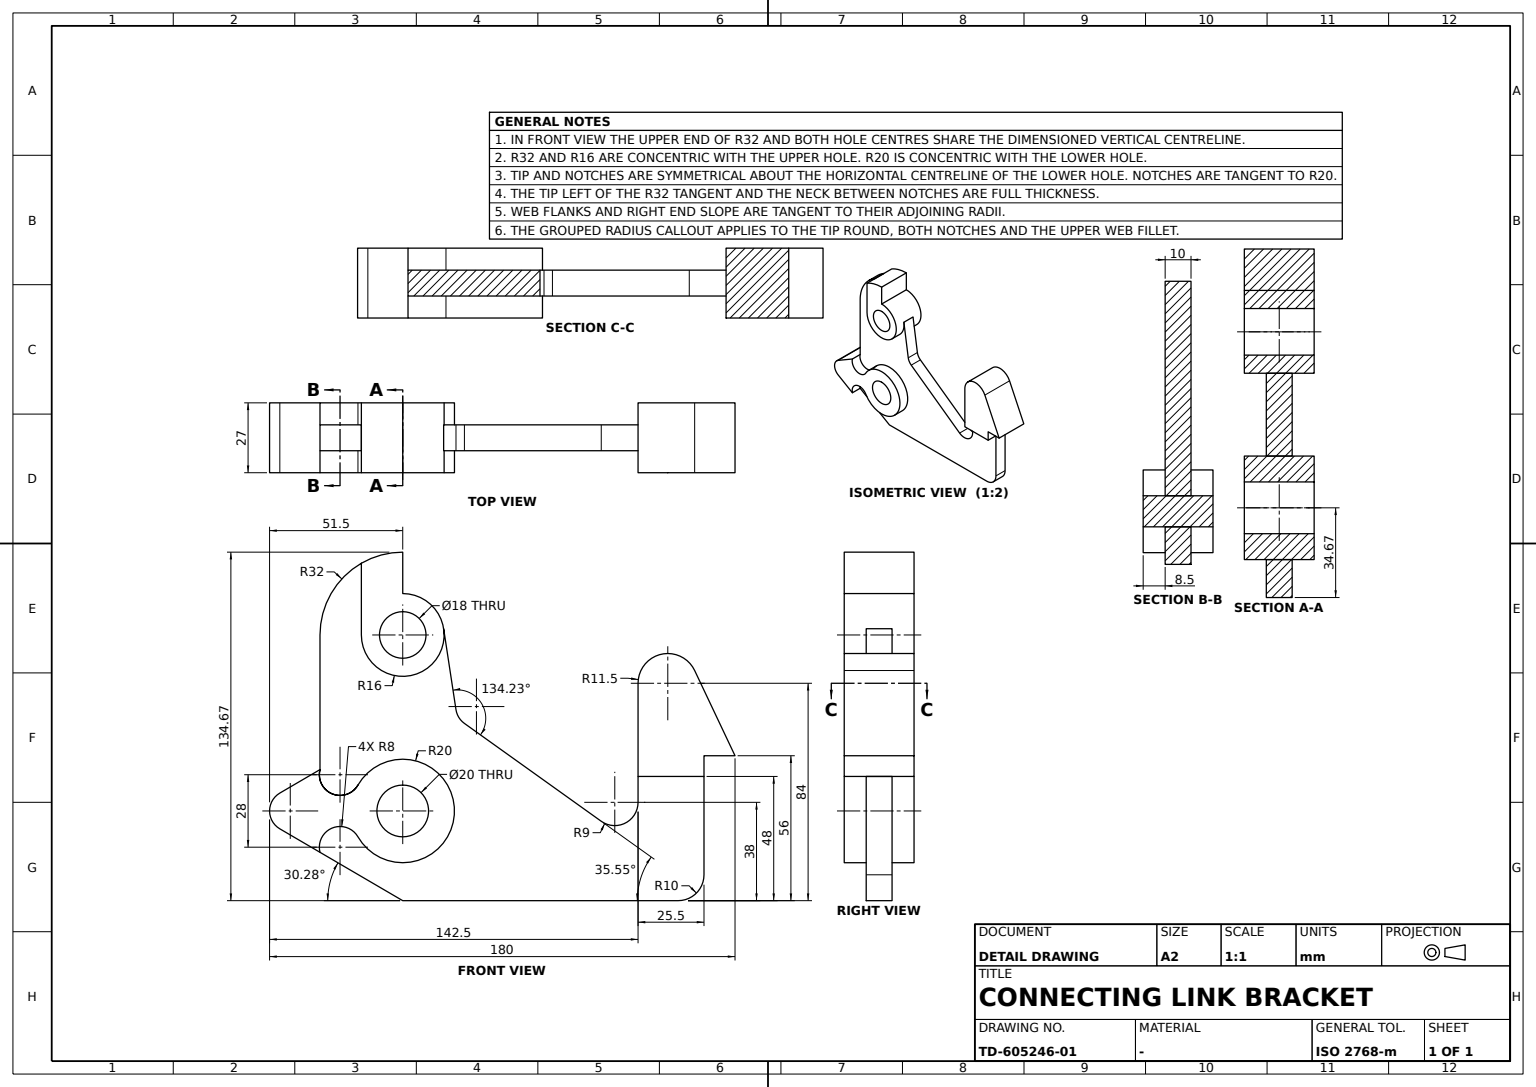
ISO-10303-21;
HEADER;
FILE_DESCRIPTION((''),'2;1');
FILE_NAME('','',(''),(''),'','','');
FILE_SCHEMA(('AUTOMOTIVE_DESIGN'));
ENDSEC;
DATA;
#1=APPLICATION_CONTEXT('');
#2=PRODUCT_CONTEXT('',#1,'mechanical');
#3=PRODUCT('','','',(#2));
#4=PRODUCT_DEFINITION_FORMATION('','',#3);
#5=PRODUCT_DEFINITION_CONTEXT('',#1,'design');
#6=PRODUCT_DEFINITION('','',#4,#5);
#7=PRODUCT_DEFINITION_SHAPE('','',#6);
#8=(LENGTH_UNIT()NAMED_UNIT(*)SI_UNIT(.MILLI.,.METRE.));
#9=(NAMED_UNIT(*)PLANE_ANGLE_UNIT()SI_UNIT($,.RADIAN.));
#10=(NAMED_UNIT(*)SI_UNIT($,.STERADIAN.)SOLID_ANGLE_UNIT());
#11=UNCERTAINTY_MEASURE_WITH_UNIT(LENGTH_MEASURE(0.005),#8,'distance_accuracy_value','');
#12=(GEOMETRIC_REPRESENTATION_CONTEXT(3)GLOBAL_UNCERTAINTY_ASSIGNED_CONTEXT((#11))GLOBAL_UNIT_ASSIGNED_CONTEXT((#8,#9,#10))REPRESENTATION_CONTEXT('',''));
#13=CARTESIAN_POINT('',(-32.,-5.,-15.979273));
#14=VERTEX_POINT('',#13);
#15=CARTESIAN_POINT('',(-32.,5.,-15.979273));
#16=VERTEX_POINT('',#15);
#17=DIRECTION('',(0.,1.,0.));
#18=VECTOR('',#17,1000.);
#19=LINE('',#13,#18);
#20=EDGE_CURVE('',#14,#16,#19,.T.);
#21=ORIENTED_EDGE('',*,*,#20,.T.);
#22=CARTESIAN_POINT('',(0.,5.,-34.665122));
#23=VERTEX_POINT('',#22);
#24=DIRECTION('',(0.863553516,0.,-0.504257201));
#25=VECTOR('',#24,1000.);
#26=LINE('',#15,#25);
#27=EDGE_CURVE('',#16,#23,#26,.T.);
#28=ORIENTED_EDGE('',*,*,#27,.T.);
#29=CARTESIAN_POINT('',(0.,-5.,-34.665122));
#30=VERTEX_POINT('',#29);
#31=LINE('',#29,#18);
#32=EDGE_CURVE('',#30,#23,#31,.T.);
#33=ORIENTED_EDGE('',*,*,#32,.F.);
#34=LINE('',#13,#25);
#35=EDGE_CURVE('',#14,#30,#34,.T.);
#36=ORIENTED_EDGE('',*,*,#35,.F.);
#37=EDGE_LOOP('',(#21,#28,#33,#36));
#38=FACE_BOUND('',#37,.T.);
#39=DIRECTION('',(0.504257201,0.,0.863553516));
#40=AXIS2_PLACEMENT_3D('',#13,#39,#24);
#41=PLANE('',#40);
#42=ADVANCED_FACE('',(#38),#41,.F.);
#43=CARTESIAN_POINT('',(20.591569,5.,39.127932));
#44=VERTEX_POINT('',#43);
#45=CARTESIAN_POINT('',(15.816862,5.,70.41389));
#46=VERTEX_POINT('',#45);
#47=DIRECTION('',(-0.150868155,0.,0.988553893));
#48=VECTOR('',#47,1000.);
#49=LINE('',#43,#48);
#50=EDGE_CURVE('',#44,#46,#49,.T.);
#51=ORIENTED_EDGE('',*,*,#50,.T.);
#52=CARTESIAN_POINT('',(15.816862,-5.,70.41389));
#53=VERTEX_POINT('',#52);
#54=LINE('',#52,#18);
#55=EDGE_CURVE('',#53,#46,#54,.T.);
#56=ORIENTED_EDGE('',*,*,#55,.F.);
#57=CARTESIAN_POINT('',(20.591569,-5.,39.127932));
#58=VERTEX_POINT('',#57);
#59=LINE('',#57,#48);
#60=EDGE_CURVE('',#58,#53,#59,.T.);
#61=ORIENTED_EDGE('',*,*,#60,.F.);
#62=LINE('',#57,#18);
#63=EDGE_CURVE('',#58,#44,#62,.T.);
#64=ORIENTED_EDGE('',*,*,#63,.T.);
#65=EDGE_LOOP('',(#51,#56,#61,#64));
#66=FACE_BOUND('',#65,.T.);
#67=DIRECTION('',(-0.988553893,0.,-0.150868155));
#68=AXIS2_PLACEMENT_3D('',#57,#67,#47);
#69=PLANE('',#68);
#70=ADVANCED_FACE('',(#66),#69,.F.);
#71=CARTESIAN_POINT('',(91.,-5.,3.334878));
#72=VERTEX_POINT('',#71);
#73=CARTESIAN_POINT('',(91.,5.,3.334878));
#74=VERTEX_POINT('',#73);
#75=LINE('',#71,#18);
#76=EDGE_CURVE('',#72,#74,#75,.T.);
#77=ORIENTED_EDGE('',*,*,#76,.F.);
#78=CARTESIAN_POINT('',(91.,-5.,13.334878));
#79=VERTEX_POINT('',#78);
#80=DIRECTION('',(0.,0.,-1.));
#81=VECTOR('',#80,1000.);
#82=LINE('',#78,#81);
#83=EDGE_CURVE('',#79,#72,#82,.T.);
#84=ORIENTED_EDGE('',*,*,#83,.F.);
#85=CARTESIAN_POINT('',(91.,5.,13.334878));
#86=VERTEX_POINT('',#85);
#87=LINE('',#78,#18);
#88=EDGE_CURVE('',#79,#86,#87,.T.);
#89=ORIENTED_EDGE('',*,*,#88,.T.);
#90=LINE('',#85,#81);
#91=EDGE_CURVE('',#86,#74,#90,.T.);
#92=ORIENTED_EDGE('',*,*,#91,.T.);
#93=EDGE_LOOP('',(#77,#84,#89,#92));
#94=FACE_BOUND('',#93,.T.);
#95=DIRECTION('',(1.,0.,0.));
#96=AXIS2_PLACEMENT_3D('',#78,#95,#80);
#97=PLANE('',#96);
#98=ADVANCED_FACE('',(#94),#97,.F.);
#99=CARTESIAN_POINT('',(0.,-5.,-20.));
#100=VERTEX_POINT('',#99);
#101=CARTESIAN_POINT('',(-17.320508,-5.,-10.));
#102=VERTEX_POINT('',#101);
#103=CARTESIAN_POINT('',(0.,-5.,0.));
#104=AXIS2_PLACEMENT_3D('',#103,#17,#95);
#105=CIRCLE('',#104,20.);
#106=EDGE_CURVE('',#100,#102,#105,.T.);
#107=ORIENTED_EDGE('',*,*,#106,.F.);
#108=CARTESIAN_POINT('',(0.,5.,-20.));
#109=VERTEX_POINT('',#108);
#110=LINE('',#99,#18);
#111=EDGE_CURVE('',#100,#109,#110,.T.);
#112=ORIENTED_EDGE('',*,*,#111,.T.);
#113=CARTESIAN_POINT('',(-17.320508,5.,-10.));
#114=VERTEX_POINT('',#113);
#115=CARTESIAN_POINT('',(0.,5.,0.));
#116=AXIS2_PLACEMENT_3D('',#115,#17,#95);
#117=CIRCLE('',#116,20.);
#118=EDGE_CURVE('',#109,#114,#117,.T.);
#119=ORIENTED_EDGE('',*,*,#118,.T.);
#120=LINE('',#101,#18);
#121=EDGE_CURVE('',#102,#114,#120,.T.);
#122=ORIENTED_EDGE('',*,*,#121,.F.);
#123=EDGE_LOOP('',(#107,#112,#119,#122));
#124=FACE_BOUND('',#123,.T.);
#125=DIRECTION('',(0.,0.,1.));
#126=AXIS2_PLACEMENT_3D('',#103,#17,#125);
#127=CYLINDRICAL_SURFACE('',#126,20.);
#128=ADVANCED_FACE('',(#124),#127,.F.);
#129=ORIENTED_EDGE('',*,*,#55,.T.);
#130=CARTESIAN_POINT('',(-16.,5.,68.));
#131=VERTEX_POINT('',#130);
#132=CARTESIAN_POINT('',(0.,5.,68.));
#133=AXIS2_PLACEMENT_3D('',#132,#17,#95);
#134=CIRCLE('',#133,16.);
#135=EDGE_CURVE('',#46,#131,#134,.T.);
#136=ORIENTED_EDGE('',*,*,#135,.T.);
#137=CARTESIAN_POINT('',(-16.,-5.,68.));
#138=VERTEX_POINT('',#137);
#139=LINE('',#137,#18);
#140=EDGE_CURVE('',#138,#131,#139,.T.);
#141=ORIENTED_EDGE('',*,*,#140,.F.);
#142=CARTESIAN_POINT('',(0.,-5.,68.));
#143=AXIS2_PLACEMENT_3D('',#142,#17,#95);
#144=CIRCLE('',#143,16.);
#145=EDGE_CURVE('',#53,#138,#144,.T.);
#146=ORIENTED_EDGE('',*,*,#145,.F.);
#147=EDGE_LOOP('',(#129,#136,#141,#146));
#148=FACE_BOUND('',#147,.T.);
#149=AXIS2_PLACEMENT_3D('',#142,#17,#125);
#150=CYLINDRICAL_SURFACE('',#149,16.);
#151=ADVANCED_FACE('',(#148),#150,.F.);
#152=CARTESIAN_POINT('',(23.848904,-5.,33.82586));
#153=VERTEX_POINT('',#152);
#154=CARTESIAN_POINT('',(23.848904,5.,33.82586));
#155=VERTEX_POINT('',#154);
#156=LINE('',#152,#18);
#157=EDGE_CURVE('',#153,#155,#156,.T.);
#158=ORIENTED_EDGE('',*,*,#157,.F.);
#159=CARTESIAN_POINT('',(76.767517,-5.,-3.987767));
#160=VERTEX_POINT('',#159);
#161=DIRECTION('',(-0.813627157,0.,0.581387005));
#162=VECTOR('',#161,1000.);
#163=LINE('',#159,#162);
#164=EDGE_CURVE('',#160,#153,#163,.T.);
#165=ORIENTED_EDGE('',*,*,#164,.F.);
#166=CARTESIAN_POINT('',(76.767517,5.,-3.987767));
#167=VERTEX_POINT('',#166);
#168=LINE('',#159,#18);
#169=EDGE_CURVE('',#160,#167,#168,.T.);
#170=ORIENTED_EDGE('',*,*,#169,.T.);
#171=LINE('',#166,#162);
#172=EDGE_CURVE('',#167,#155,#171,.T.);
#173=ORIENTED_EDGE('',*,*,#172,.T.);
#174=EDGE_LOOP('',(#158,#165,#170,#173));
#175=FACE_BOUND('',#174,.T.);
#176=DIRECTION('',(-0.581387005,0.,-0.813627157));
#177=AXIS2_PLACEMENT_3D('',#159,#176,#161);
#178=PLANE('',#177);
#179=ADVANCED_FACE('',(#175),#178,.F.);
#180=CARTESIAN_POINT('',(-16.,5.,95.712813));
#181=VERTEX_POINT('',#180);
#182=VECTOR('',#125,1000.);
#183=LINE('',#130,#182);
#184=EDGE_CURVE('',#131,#181,#183,.T.);
#185=ORIENTED_EDGE('',*,*,#184,.T.);
#186=CARTESIAN_POINT('',(-16.,-5.,95.712813));
#187=VERTEX_POINT('',#186);
#188=LINE('',#186,#18);
#189=EDGE_CURVE('',#187,#181,#188,.T.);
#190=ORIENTED_EDGE('',*,*,#189,.F.);
#191=LINE('',#137,#182);
#192=EDGE_CURVE('',#138,#187,#191,.T.);
#193=ORIENTED_EDGE('',*,*,#192,.F.);
#194=ORIENTED_EDGE('',*,*,#140,.T.);
#195=EDGE_LOOP('',(#185,#190,#193,#194));
#196=FACE_BOUND('',#195,.T.);
#197=DIRECTION('',(-1.,0.,0.));
#198=AXIS2_PLACEMENT_3D('',#137,#197,#125);
#199=PLANE('',#198);
#200=ADVANCED_FACE('',(#196),#199,.F.);
#201=CARTESIAN_POINT('',(-24.248711,-5.,-6.));
#202=VERTEX_POINT('',#201);
#203=CARTESIAN_POINT('',(-24.248711,5.,-6.));
#204=VERTEX_POINT('',#203);
#205=LINE('',#201,#18);
#206=EDGE_CURVE('',#202,#204,#205,.T.);
#207=ORIENTED_EDGE('',*,*,#206,.F.);
#208=CARTESIAN_POINT('',(-24.248711,-5.,-14.));
#209=DIRECTION('',(0.,-1.,0.));
#210=AXIS2_PLACEMENT_3D('',#208,#209,#95);
#211=CIRCLE('',#210,8.);
#212=EDGE_CURVE('',#102,#202,#211,.T.);
#213=ORIENTED_EDGE('',*,*,#212,.F.);
#214=ORIENTED_EDGE('',*,*,#121,.T.);
#215=CARTESIAN_POINT('',(-24.248711,5.,-14.));
#216=AXIS2_PLACEMENT_3D('',#215,#209,#95);
#217=CIRCLE('',#216,8.);
#218=EDGE_CURVE('',#114,#204,#217,.T.);
#219=ORIENTED_EDGE('',*,*,#218,.T.);
#220=EDGE_LOOP('',(#207,#213,#214,#219));
#221=FACE_BOUND('',#220,.T.);
#222=AXIS2_PLACEMENT_3D('',#208,#17,#125);
#223=CYLINDRICAL_SURFACE('',#222,8.);
#224=ADVANCED_FACE('',(#221),#223,.T.);
#225=CARTESIAN_POINT('',(-32.,-5.,15.979273));
#226=VERTEX_POINT('',#225);
#227=CARTESIAN_POINT('',(-32.,5.,15.979273));
#228=VERTEX_POINT('',#227);
#229=LINE('',#225,#18);
#230=EDGE_CURVE('',#226,#228,#229,.T.);
#231=ORIENTED_EDGE('',*,*,#230,.F.);
#232=CARTESIAN_POINT('',(-32.,-5.,68.));
#233=VERTEX_POINT('',#232);
#234=LINE('',#232,#81);
#235=EDGE_CURVE('',#233,#226,#234,.T.);
#236=ORIENTED_EDGE('',*,*,#235,.F.);
#237=CARTESIAN_POINT('',(-32.,5.,68.));
#238=VERTEX_POINT('',#237);
#239=LINE('',#232,#18);
#240=EDGE_CURVE('',#233,#238,#239,.T.);
#241=ORIENTED_EDGE('',*,*,#240,.T.);
#242=LINE('',#237,#81);
#243=EDGE_CURVE('',#238,#228,#242,.T.);
#244=ORIENTED_EDGE('',*,*,#243,.T.);
#245=EDGE_LOOP('',(#231,#236,#241,#244));
#246=FACE_BOUND('',#245,.T.);
#247=AXIS2_PLACEMENT_3D('',#232,#95,#80);
#248=PLANE('',#247);
#249=ADVANCED_FACE('',(#246),#248,.F.);
#250=CARTESIAN_POINT('',(-17.320508,-5.,10.));
#251=VERTEX_POINT('',#250);
#252=CARTESIAN_POINT('',(-24.248711,-5.,14.));
#253=AXIS2_PLACEMENT_3D('',#252,#209,#95);
#254=CIRCLE('',#253,8.);
#255=EDGE_CURVE('',#226,#251,#254,.T.);
#256=ORIENTED_EDGE('',*,*,#255,.F.);
#257=ORIENTED_EDGE('',*,*,#230,.T.);
#258=CARTESIAN_POINT('',(-17.320508,5.,10.));
#259=VERTEX_POINT('',#258);
#260=CARTESIAN_POINT('',(-24.248711,5.,14.));
#261=AXIS2_PLACEMENT_3D('',#260,#209,#95);
#262=CIRCLE('',#261,8.);
#263=EDGE_CURVE('',#228,#259,#262,.T.);
#264=ORIENTED_EDGE('',*,*,#263,.T.);
#265=LINE('',#250,#18);
#266=EDGE_CURVE('',#251,#259,#265,.T.);
#267=ORIENTED_EDGE('',*,*,#266,.F.);
#268=EDGE_LOOP('',(#256,#257,#264,#267));
#269=FACE_BOUND('',#268,.T.);
#270=AXIS2_PLACEMENT_3D('',#252,#17,#125);
#271=CYLINDRICAL_SURFACE('',#270,8.);
#272=ADVANCED_FACE('',(#269),#271,.T.);
#273=ORIENTED_EDGE('',*,*,#157,.T.);
#274=CARTESIAN_POINT('',(28.5,5.,40.334878));
#275=AXIS2_PLACEMENT_3D('',#274,#17,#95);
#276=CIRCLE('',#275,8.);
#277=EDGE_CURVE('',#155,#44,#276,.T.);
#278=ORIENTED_EDGE('',*,*,#277,.T.);
#279=ORIENTED_EDGE('',*,*,#63,.F.);
#280=CARTESIAN_POINT('',(28.5,-5.,40.334878));
#281=AXIS2_PLACEMENT_3D('',#280,#17,#95);
#282=CIRCLE('',#281,8.);
#283=EDGE_CURVE('',#153,#58,#282,.T.);
#284=ORIENTED_EDGE('',*,*,#283,.F.);
#285=EDGE_LOOP('',(#273,#278,#279,#284));
#286=FACE_BOUND('',#285,.T.);
#287=AXIS2_PLACEMENT_3D('',#280,#17,#125);
#288=CYLINDRICAL_SURFACE('',#287,8.);
#289=ADVANCED_FACE('',(#286),#288,.F.);
#290=ORIENTED_EDGE('',*,*,#240,.F.);
#291=AXIS2_PLACEMENT_3D('',#142,#209,#95);
#292=CIRCLE('',#291,32.);
#293=EDGE_CURVE('',#187,#233,#292,.T.);
#294=ORIENTED_EDGE('',*,*,#293,.F.);
#295=ORIENTED_EDGE('',*,*,#189,.T.);
#296=AXIS2_PLACEMENT_3D('',#132,#209,#95);
#297=CIRCLE('',#296,32.);
#298=EDGE_CURVE('',#181,#238,#297,.T.);
#299=ORIENTED_EDGE('',*,*,#298,.T.);
#300=EDGE_LOOP('',(#290,#294,#295,#299));
#301=FACE_BOUND('',#300,.T.);
#302=CYLINDRICAL_SURFACE('',#149,32.);
#303=ADVANCED_FACE('',(#301),#302,.T.);
#304=CARTESIAN_POINT('',(116.5,-5.,13.334878));
#305=VERTEX_POINT('',#304);
#306=CARTESIAN_POINT('',(116.5,5.,13.334878));
#307=VERTEX_POINT('',#306);
#308=LINE('',#304,#18);
#309=EDGE_CURVE('',#305,#307,#308,.T.);
#310=ORIENTED_EDGE('',*,*,#309,.F.);
#311=CARTESIAN_POINT('',(116.5,-5.,-24.665122));
#312=VERTEX_POINT('',#311);
#313=LINE('',#311,#182);
#314=EDGE_CURVE('',#312,#305,#313,.T.);
#315=ORIENTED_EDGE('',*,*,#314,.F.);
#316=CARTESIAN_POINT('',(116.5,5.,-24.665122));
#317=VERTEX_POINT('',#316);
#318=LINE('',#311,#18);
#319=EDGE_CURVE('',#312,#317,#318,.T.);
#320=ORIENTED_EDGE('',*,*,#319,.T.);
#321=LINE('',#316,#182);
#322=EDGE_CURVE('',#317,#307,#321,.T.);
#323=ORIENTED_EDGE('',*,*,#322,.T.);
#324=EDGE_LOOP('',(#310,#315,#320,#323));
#325=FACE_BOUND('',#324,.T.);
#326=AXIS2_PLACEMENT_3D('',#311,#197,#125);
#327=PLANE('',#326);
#328=ADVANCED_FACE('',(#325),#327,.F.);
#329=ORIENTED_EDGE('',*,*,#32,.T.);
#330=CARTESIAN_POINT('',(106.5,5.,-34.665122));
#331=VERTEX_POINT('',#330);
#332=VECTOR('',#95,1000.);
#333=LINE('',#22,#332);
#334=EDGE_CURVE('',#23,#331,#333,.T.);
#335=ORIENTED_EDGE('',*,*,#334,.T.);
#336=CARTESIAN_POINT('',(106.5,-5.,-34.665122));
#337=VERTEX_POINT('',#336);
#338=LINE('',#336,#18);
#339=EDGE_CURVE('',#337,#331,#338,.T.);
#340=ORIENTED_EDGE('',*,*,#339,.F.);
#341=LINE('',#29,#332);
#342=EDGE_CURVE('',#30,#337,#341,.T.);
#343=ORIENTED_EDGE('',*,*,#342,.F.);
#344=EDGE_LOOP('',(#329,#335,#340,#343));
#345=FACE_BOUND('',#344,.T.);
#346=AXIS2_PLACEMENT_3D('',#29,#125,#95);
#347=PLANE('',#346);
#348=ADVANCED_FACE('',(#345),#347,.F.);
#349=ORIENTED_EDGE('',*,*,#135,.F.);
#350=ORIENTED_EDGE('',*,*,#50,.F.);
#351=ORIENTED_EDGE('',*,*,#277,.F.);
#352=ORIENTED_EDGE('',*,*,#172,.F.);
#353=CARTESIAN_POINT('',(82.,5.,3.334878));
#354=AXIS2_PLACEMENT_3D('',#353,#17,#95);
#355=CIRCLE('',#354,9.);
#356=EDGE_CURVE('',#74,#167,#355,.T.);
#357=ORIENTED_EDGE('',*,*,#356,.F.);
#358=ORIENTED_EDGE('',*,*,#91,.F.);
#359=VECTOR('',#197,1000.);
#360=LINE('',#306,#359);
#361=EDGE_CURVE('',#307,#86,#360,.T.);
#362=ORIENTED_EDGE('',*,*,#361,.F.);
#363=ORIENTED_EDGE('',*,*,#322,.F.);
#364=CARTESIAN_POINT('',(106.5,5.,-24.665122));
#365=AXIS2_PLACEMENT_3D('',#364,#209,#95);
#366=CIRCLE('',#365,10.);
#367=EDGE_CURVE('',#331,#317,#366,.T.);
#368=ORIENTED_EDGE('',*,*,#367,.F.);
#369=ORIENTED_EDGE('',*,*,#334,.F.);
#370=ORIENTED_EDGE('',*,*,#27,.F.);
#371=EDGE_CURVE('',#204,#16,#217,.T.);
#372=ORIENTED_EDGE('',*,*,#371,.F.);
#373=ORIENTED_EDGE('',*,*,#218,.F.);
#374=ORIENTED_EDGE('',*,*,#118,.F.);
#375=CARTESIAN_POINT('',(0.,5.,20.));
#376=VERTEX_POINT('',#375);
#377=EDGE_CURVE('',#376,#109,#117,.T.);
#378=ORIENTED_EDGE('',*,*,#377,.F.);
#379=EDGE_CURVE('',#259,#376,#117,.T.);
#380=ORIENTED_EDGE('',*,*,#379,.F.);
#381=ORIENTED_EDGE('',*,*,#263,.F.);
#382=ORIENTED_EDGE('',*,*,#243,.F.);
#383=ORIENTED_EDGE('',*,*,#298,.F.);
#384=ORIENTED_EDGE('',*,*,#184,.F.);
#385=EDGE_LOOP('',(#349,#350,#351,#352,#357,#358,#362,#363,#368,#369,#370,#372,#373,#374,#378,#380,#381,#382,#383,#384));
#386=FACE_BOUND('',#385,.T.);
#387=AXIS2_PLACEMENT_3D('',#215,#209,#80);
#388=PLANE('',#387);
#389=ADVANCED_FACE('',(#386),#388,.F.);
#390=CARTESIAN_POINT('',(0.,-5.,20.));
#391=VERTEX_POINT('',#390);
#392=LINE('',#390,#18);
#393=EDGE_CURVE('',#391,#376,#392,.T.);
#394=ORIENTED_EDGE('',*,*,#393,.F.);
#395=EDGE_CURVE('',#251,#391,#105,.T.);
#396=ORIENTED_EDGE('',*,*,#395,.F.);
#397=ORIENTED_EDGE('',*,*,#266,.T.);
#398=ORIENTED_EDGE('',*,*,#379,.T.);
#399=EDGE_LOOP('',(#394,#396,#397,#398));
#400=FACE_BOUND('',#399,.T.);
#401=ADVANCED_FACE('',(#400),#127,.F.);
#402=ORIENTED_EDGE('',*,*,#88,.F.);
#403=LINE('',#304,#359);
#404=EDGE_CURVE('',#305,#79,#403,.T.);
#405=ORIENTED_EDGE('',*,*,#404,.F.);
#406=ORIENTED_EDGE('',*,*,#309,.T.);
#407=ORIENTED_EDGE('',*,*,#361,.T.);
#408=EDGE_LOOP('',(#402,#405,#406,#407));
#409=FACE_BOUND('',#408,.T.);
#410=AXIS2_PLACEMENT_3D('',#304,#80,#197);
#411=PLANE('',#410);
#412=ADVANCED_FACE('',(#409),#411,.F.);
#413=ORIENTED_EDGE('',*,*,#393,.T.);
#414=ORIENTED_EDGE('',*,*,#377,.T.);
#415=ORIENTED_EDGE('',*,*,#111,.F.);
#416=EDGE_CURVE('',#391,#100,#105,.T.);
#417=ORIENTED_EDGE('',*,*,#416,.F.);
#418=EDGE_LOOP('',(#413,#414,#415,#417));
#419=FACE_BOUND('',#418,.T.);
#420=ADVANCED_FACE('',(#419),#127,.F.);
#421=ORIENTED_EDGE('',*,*,#356,.T.);
#422=ORIENTED_EDGE('',*,*,#169,.F.);
#423=CARTESIAN_POINT('',(82.,-5.,3.334878));
#424=AXIS2_PLACEMENT_3D('',#423,#17,#95);
#425=CIRCLE('',#424,9.);
#426=EDGE_CURVE('',#72,#160,#425,.T.);
#427=ORIENTED_EDGE('',*,*,#426,.F.);
#428=ORIENTED_EDGE('',*,*,#76,.T.);
#429=EDGE_LOOP('',(#421,#422,#427,#428));
#430=FACE_BOUND('',#429,.T.);
#431=AXIS2_PLACEMENT_3D('',#423,#17,#125);
#432=CYLINDRICAL_SURFACE('',#431,9.);
#433=ADVANCED_FACE('',(#430),#432,.F.);
#434=ORIENTED_EDGE('',*,*,#367,.T.);
#435=ORIENTED_EDGE('',*,*,#319,.F.);
#436=CARTESIAN_POINT('',(106.5,-5.,-24.665122));
#437=AXIS2_PLACEMENT_3D('',#436,#209,#95);
#438=CIRCLE('',#437,10.);
#439=EDGE_CURVE('',#337,#312,#438,.T.);
#440=ORIENTED_EDGE('',*,*,#439,.F.);
#441=ORIENTED_EDGE('',*,*,#339,.T.);
#442=EDGE_LOOP('',(#434,#435,#440,#441));
#443=FACE_BOUND('',#442,.T.);
#444=AXIS2_PLACEMENT_3D('',#436,#17,#125);
#445=CYLINDRICAL_SURFACE('',#444,10.);
#446=ADVANCED_FACE('',(#443),#445,.T.);
#447=ORIENTED_EDGE('',*,*,#20,.F.);
#448=EDGE_CURVE('',#202,#14,#211,.T.);
#449=ORIENTED_EDGE('',*,*,#448,.F.);
#450=ORIENTED_EDGE('',*,*,#206,.T.);
#451=ORIENTED_EDGE('',*,*,#371,.T.);
#452=EDGE_LOOP('',(#447,#449,#450,#451));
#453=FACE_BOUND('',#452,.T.);
#454=ADVANCED_FACE('',(#453),#223,.T.);
#455=ORIENTED_EDGE('',*,*,#164,.T.);
#456=ORIENTED_EDGE('',*,*,#283,.T.);
#457=ORIENTED_EDGE('',*,*,#60,.T.);
#458=ORIENTED_EDGE('',*,*,#145,.T.);
#459=ORIENTED_EDGE('',*,*,#192,.T.);
#460=ORIENTED_EDGE('',*,*,#293,.T.);
#461=ORIENTED_EDGE('',*,*,#235,.T.);
#462=ORIENTED_EDGE('',*,*,#255,.T.);
#463=ORIENTED_EDGE('',*,*,#395,.T.);
#464=ORIENTED_EDGE('',*,*,#416,.T.);
#465=ORIENTED_EDGE('',*,*,#106,.T.);
#466=ORIENTED_EDGE('',*,*,#212,.T.);
#467=ORIENTED_EDGE('',*,*,#448,.T.);
#468=ORIENTED_EDGE('',*,*,#35,.T.);
#469=ORIENTED_EDGE('',*,*,#342,.T.);
#470=ORIENTED_EDGE('',*,*,#439,.T.);
#471=ORIENTED_EDGE('',*,*,#314,.T.);
#472=ORIENTED_EDGE('',*,*,#404,.T.);
#473=ORIENTED_EDGE('',*,*,#83,.T.);
#474=ORIENTED_EDGE('',*,*,#426,.T.);
#475=EDGE_LOOP('',(#455,#456,#457,#458,#459,#460,#461,#462,#463,#464,#465,#466,#467,#468,#469,#470,#471,#472,#473,#474));
#476=FACE_BOUND('',#475,.T.);
#477=AXIS2_PLACEMENT_3D('',#208,#209,#80);
#478=PLANE('',#477);
#479=ADVANCED_FACE('',(#476),#478,.T.);
#480=CLOSED_SHELL('',(#42,#70,#98,#128,#151,#179,#200,#224,#249,#272,#289,#303,#328,#348,#389,#401,#412,#420,#433,#446,#454,#479));
#481=MANIFOLD_SOLID_BREP('',#480);
#482=CARTESIAN_POINT('',(91.,-13.5,49.334878));
#483=VERTEX_POINT('',#482);
#484=CARTESIAN_POINT('',(91.,13.5,49.334878));
#485=VERTEX_POINT('',#484);
#486=LINE('',#482,#18);
#487=EDGE_CURVE('',#483,#485,#486,.T.);
#488=ORIENTED_EDGE('',*,*,#487,.F.);
#489=CARTESIAN_POINT('',(102.5,-13.5,60.834878));
#490=VERTEX_POINT('',#489);
#491=CARTESIAN_POINT('',(102.5,-13.5,49.334878));
#492=AXIS2_PLACEMENT_3D('',#491,#209,#95);
#493=CIRCLE('',#492,11.5);
#494=EDGE_CURVE('',#490,#483,#493,.T.);
#495=ORIENTED_EDGE('',*,*,#494,.F.);
#496=CARTESIAN_POINT('',(102.5,13.5,60.834878));
#497=VERTEX_POINT('',#496);
#498=LINE('',#489,#18);
#499=EDGE_CURVE('',#490,#497,#498,.T.);
#500=ORIENTED_EDGE('',*,*,#499,.T.);
#501=CARTESIAN_POINT('',(102.5,13.5,49.334878));
#502=AXIS2_PLACEMENT_3D('',#501,#209,#95);
#503=CIRCLE('',#502,11.5);
#504=EDGE_CURVE('',#497,#485,#503,.T.);
#505=ORIENTED_EDGE('',*,*,#504,.T.);
#506=EDGE_LOOP('',(#488,#495,#500,#505));
#507=FACE_BOUND('',#506,.T.);
#508=AXIS2_PLACEMENT_3D('',#491,#17,#125);
#509=CYLINDRICAL_SURFACE('',#508,11.5);
#510=ADVANCED_FACE('',(#507),#509,.T.);
#511=CARTESIAN_POINT('',(116.5,-13.5,13.334878));
#512=VERTEX_POINT('',#511);
#513=CARTESIAN_POINT('',(116.5,13.5,13.334878));
#514=VERTEX_POINT('',#513);
#515=LINE('',#511,#18);
#516=EDGE_CURVE('',#512,#514,#515,.T.);
#517=ORIENTED_EDGE('',*,*,#516,.F.);
#518=CARTESIAN_POINT('',(91.,-13.5,13.334878));
#519=VERTEX_POINT('',#518);
#520=LINE('',#518,#332);
#521=EDGE_CURVE('',#519,#512,#520,.T.);
#522=ORIENTED_EDGE('',*,*,#521,.F.);
#523=CARTESIAN_POINT('',(91.,13.5,13.334878));
#524=VERTEX_POINT('',#523);
#525=LINE('',#518,#18);
#526=EDGE_CURVE('',#519,#524,#525,.T.);
#527=ORIENTED_EDGE('',*,*,#526,.T.);
#528=LINE('',#523,#332);
#529=EDGE_CURVE('',#524,#514,#528,.T.);
#530=ORIENTED_EDGE('',*,*,#529,.T.);
#531=EDGE_LOOP('',(#517,#522,#527,#530));
#532=FACE_BOUND('',#531,.T.);
#533=AXIS2_PLACEMENT_3D('',#518,#125,#95);
#534=PLANE('',#533);
#535=ADVANCED_FACE('',(#532),#534,.F.);
#536=CARTESIAN_POINT('',(116.5,-13.5,21.334878));
#537=VERTEX_POINT('',#536);
#538=LINE('',#511,#182);
#539=EDGE_CURVE('',#512,#537,#538,.T.);
#540=ORIENTED_EDGE('',*,*,#539,.F.);
#541=ORIENTED_EDGE('',*,*,#516,.T.);
#542=CARTESIAN_POINT('',(116.5,13.5,21.334878));
#543=VERTEX_POINT('',#542);
#544=LINE('',#513,#182);
#545=EDGE_CURVE('',#514,#543,#544,.T.);
#546=ORIENTED_EDGE('',*,*,#545,.T.);
#547=LINE('',#536,#18);
#548=EDGE_CURVE('',#537,#543,#547,.T.);
#549=ORIENTED_EDGE('',*,*,#548,.F.);
#550=EDGE_LOOP('',(#540,#541,#546,#549));
#551=FACE_BOUND('',#550,.T.);
#552=AXIS2_PLACEMENT_3D('',#511,#197,#125);
#553=PLANE('',#552);
#554=ADVANCED_FACE('',(#551),#553,.F.);
#555=CARTESIAN_POINT('',(128.5,13.5,21.334878));
#556=VERTEX_POINT('',#555);
#557=CARTESIAN_POINT('',(112.89153,13.5,54.260941));
#558=VERTEX_POINT('',#557);
#559=DIRECTION('',(-0.428353359,0.,0.90361131));
#560=VECTOR('',#559,1000.);
#561=LINE('',#555,#560);
#562=EDGE_CURVE('',#556,#558,#561,.T.);
#563=ORIENTED_EDGE('',*,*,#562,.T.);
#564=CARTESIAN_POINT('',(112.89153,-13.5,54.260941));
#565=VERTEX_POINT('',#564);
#566=LINE('',#564,#18);
#567=EDGE_CURVE('',#565,#558,#566,.T.);
#568=ORIENTED_EDGE('',*,*,#567,.F.);
#569=CARTESIAN_POINT('',(128.5,-13.5,21.334878));
#570=VERTEX_POINT('',#569);
#571=LINE('',#569,#560);
#572=EDGE_CURVE('',#570,#565,#571,.T.);
#573=ORIENTED_EDGE('',*,*,#572,.F.);
#574=LINE('',#569,#18);
#575=EDGE_CURVE('',#570,#556,#574,.T.);
#576=ORIENTED_EDGE('',*,*,#575,.T.);
#577=EDGE_LOOP('',(#563,#568,#573,#576));
#578=FACE_BOUND('',#577,.T.);
#579=DIRECTION('',(-0.90361131,0.,-0.428353359));
#580=AXIS2_PLACEMENT_3D('',#569,#579,#559);
#581=PLANE('',#580);
#582=ADVANCED_FACE('',(#578),#581,.F.);
#583=ORIENTED_EDGE('',*,*,#529,.F.);
#584=LINE('',#484,#81);
#585=EDGE_CURVE('',#485,#524,#584,.T.);
#586=ORIENTED_EDGE('',*,*,#585,.F.);
#587=ORIENTED_EDGE('',*,*,#504,.F.);
#588=EDGE_CURVE('',#558,#497,#503,.T.);
#589=ORIENTED_EDGE('',*,*,#588,.F.);
#590=ORIENTED_EDGE('',*,*,#562,.F.);
#591=LINE('',#542,#332);
#592=EDGE_CURVE('',#543,#556,#591,.T.);
#593=ORIENTED_EDGE('',*,*,#592,.F.);
#594=ORIENTED_EDGE('',*,*,#545,.F.);
#595=EDGE_LOOP('',(#583,#586,#587,#589,#590,#593,#594));
#596=FACE_BOUND('',#595,.T.);
#597=AXIS2_PLACEMENT_3D('',#501,#209,#80);
#598=PLANE('',#597);
#599=ADVANCED_FACE('',(#596),#598,.F.);
#600=ORIENTED_EDGE('',*,*,#575,.F.);
#601=LINE('',#536,#332);
#602=EDGE_CURVE('',#537,#570,#601,.T.);
#603=ORIENTED_EDGE('',*,*,#602,.F.);
#604=ORIENTED_EDGE('',*,*,#548,.T.);
#605=ORIENTED_EDGE('',*,*,#592,.T.);
#606=EDGE_LOOP('',(#600,#603,#604,#605));
#607=FACE_BOUND('',#606,.T.);
#608=AXIS2_PLACEMENT_3D('',#536,#125,#95);
#609=PLANE('',#608);
#610=ADVANCED_FACE('',(#607),#609,.F.);
#611=ORIENTED_EDGE('',*,*,#499,.F.);
#612=EDGE_CURVE('',#565,#490,#493,.T.);
#613=ORIENTED_EDGE('',*,*,#612,.F.);
#614=ORIENTED_EDGE('',*,*,#567,.T.);
#615=ORIENTED_EDGE('',*,*,#588,.T.);
#616=EDGE_LOOP('',(#611,#613,#614,#615));
#617=FACE_BOUND('',#616,.T.);
#618=ADVANCED_FACE('',(#617),#509,.T.);
#619=LINE('',#482,#81);
#620=EDGE_CURVE('',#483,#519,#619,.T.);
#621=ORIENTED_EDGE('',*,*,#620,.F.);
#622=ORIENTED_EDGE('',*,*,#487,.T.);
#623=ORIENTED_EDGE('',*,*,#585,.T.);
#624=ORIENTED_EDGE('',*,*,#526,.F.);
#625=EDGE_LOOP('',(#621,#622,#623,#624));
#626=FACE_BOUND('',#625,.T.);
#627=AXIS2_PLACEMENT_3D('',#482,#95,#80);
#628=PLANE('',#627);
#629=ADVANCED_FACE('',(#626),#628,.F.);
#630=ORIENTED_EDGE('',*,*,#602,.T.);
#631=ORIENTED_EDGE('',*,*,#572,.T.);
#632=ORIENTED_EDGE('',*,*,#612,.T.);
#633=ORIENTED_EDGE('',*,*,#494,.T.);
#634=ORIENTED_EDGE('',*,*,#620,.T.);
#635=ORIENTED_EDGE('',*,*,#521,.T.);
#636=ORIENTED_EDGE('',*,*,#539,.T.);
#637=EDGE_LOOP('',(#630,#631,#632,#633,#634,#635,#636));
#638=FACE_BOUND('',#637,.T.);
#639=AXIS2_PLACEMENT_3D('',#491,#209,#80);
#640=PLANE('',#639);
#641=ADVANCED_FACE('',(#638),#640,.T.);
#642=CLOSED_SHELL('',(#510,#535,#554,#582,#599,#610,#618,#629,#641));
#643=MANIFOLD_SOLID_BREP('',#642);
#644=CARTESIAN_POINT('',(-32.,-13.5,15.979273));
#645=VERTEX_POINT('',#644);
#646=CARTESIAN_POINT('',(-32.,13.5,15.979273));
#647=VERTEX_POINT('',#646);
#648=LINE('',#644,#18);
#649=EDGE_CURVE('',#645,#647,#648,.T.);
#650=ORIENTED_EDGE('',*,*,#649,.F.);
#651=CARTESIAN_POINT('',(-17.320508,-13.5,10.));
#652=VERTEX_POINT('',#651);
#653=CARTESIAN_POINT('',(-24.248711,-13.5,14.));
#654=AXIS2_PLACEMENT_3D('',#653,#17,#95);
#655=CIRCLE('',#654,8.);
#656=EDGE_CURVE('',#652,#645,#655,.T.);
#657=ORIENTED_EDGE('',*,*,#656,.F.);
#658=CARTESIAN_POINT('',(-17.320508,13.5,10.));
#659=VERTEX_POINT('',#658);
#660=LINE('',#651,#18);
#661=EDGE_CURVE('',#652,#659,#660,.T.);
#662=ORIENTED_EDGE('',*,*,#661,.T.);
#663=CARTESIAN_POINT('',(-24.248711,13.5,14.));
#664=AXIS2_PLACEMENT_3D('',#663,#17,#95);
#665=CIRCLE('',#664,8.);
#666=EDGE_CURVE('',#659,#647,#665,.T.);
#667=ORIENTED_EDGE('',*,*,#666,.T.);
#668=EDGE_LOOP('',(#650,#657,#662,#667));
#669=FACE_BOUND('',#668,.T.);
#670=AXIS2_PLACEMENT_3D('',#653,#17,#125);
#671=CYLINDRICAL_SURFACE('',#670,8.);
#672=ADVANCED_FACE('',(#669),#671,.F.);
#673=CARTESIAN_POINT('',(0.,13.5,-10.));
#674=VERTEX_POINT('',#673);
#675=CARTESIAN_POINT('',(0.,13.5,10.));
#676=VERTEX_POINT('',#675);
#677=CARTESIAN_POINT('',(0.,13.5,0.));
#678=AXIS2_PLACEMENT_3D('',#677,#209,#95);
#679=CIRCLE('',#678,10.);
#680=EDGE_CURVE('',#674,#676,#679,.T.);
#681=ORIENTED_EDGE('',*,*,#680,.T.);
#682=EDGE_CURVE('',#676,#674,#679,.T.);
#683=ORIENTED_EDGE('',*,*,#682,.T.);
#684=EDGE_LOOP('',(#681,#683));
#685=FACE_BOUND('',#684,.T.);
#686=CARTESIAN_POINT('',(0.,13.5,-20.));
#687=VERTEX_POINT('',#686);
#688=CARTESIAN_POINT('',(0.,13.5,20.));
#689=VERTEX_POINT('',#688);
#690=CIRCLE('',#678,20.);
#691=EDGE_CURVE('',#687,#689,#690,.T.);
#692=ORIENTED_EDGE('',*,*,#691,.F.);
#693=CARTESIAN_POINT('',(-17.320508,13.5,-10.));
#694=VERTEX_POINT('',#693);
#695=EDGE_CURVE('',#694,#687,#690,.T.);
#696=ORIENTED_EDGE('',*,*,#695,.F.);
#697=CARTESIAN_POINT('',(-24.248711,13.5,-6.));
#698=VERTEX_POINT('',#697);
#699=CARTESIAN_POINT('',(-24.248711,13.5,-14.));
#700=AXIS2_PLACEMENT_3D('',#699,#17,#95);
#701=CIRCLE('',#700,8.);
#702=EDGE_CURVE('',#698,#694,#701,.T.);
#703=ORIENTED_EDGE('',*,*,#702,.F.);
#704=CARTESIAN_POINT('',(-32.,13.5,-15.979273));
#705=VERTEX_POINT('',#704);
#706=EDGE_CURVE('',#705,#698,#701,.T.);
#707=ORIENTED_EDGE('',*,*,#706,.F.);
#708=CARTESIAN_POINT('',(-47.534058,13.5,-6.908428));
#709=VERTEX_POINT('',#708);
#710=LINE('',#708,#25);
#711=EDGE_CURVE('',#709,#705,#710,.T.);
#712=ORIENTED_EDGE('',*,*,#711,.F.);
#713=CARTESIAN_POINT('',(-47.534058,13.5,6.908428));
#714=VERTEX_POINT('',#713);
#715=CARTESIAN_POINT('',(-43.5,13.5,0.));
#716=AXIS2_PLACEMENT_3D('',#715,#209,#95);
#717=CIRCLE('',#716,8.);
#718=EDGE_CURVE('',#714,#709,#717,.T.);
#719=ORIENTED_EDGE('',*,*,#718,.F.);
#720=DIRECTION('',(-0.863553516,0.,-0.504257201));
#721=VECTOR('',#720,1000.);
#722=LINE('',#646,#721);
#723=EDGE_CURVE('',#647,#714,#722,.T.);
#724=ORIENTED_EDGE('',*,*,#723,.F.);
#725=ORIENTED_EDGE('',*,*,#666,.F.);
#726=EDGE_CURVE('',#689,#659,#690,.T.);
#727=ORIENTED_EDGE('',*,*,#726,.F.);
#728=EDGE_LOOP('',(#692,#696,#703,#707,#712,#719,#724,#725,#727));
#729=FACE_BOUND('',#728,.T.);
#730=AXIS2_PLACEMENT_3D('',#715,#209,#80);
#731=PLANE('',#730);
#732=ADVANCED_FACE('',(#685,#729),#731,.F.);
#733=CARTESIAN_POINT('',(-47.534058,-13.5,6.908428));
#734=VERTEX_POINT('',#733);
#735=LINE('',#733,#18);
#736=EDGE_CURVE('',#734,#714,#735,.T.);
#737=ORIENTED_EDGE('',*,*,#736,.T.);
#738=ORIENTED_EDGE('',*,*,#718,.T.);
#739=CARTESIAN_POINT('',(-47.534058,-13.5,-6.908428));
#740=VERTEX_POINT('',#739);
#741=LINE('',#739,#18);
#742=EDGE_CURVE('',#740,#709,#741,.T.);
#743=ORIENTED_EDGE('',*,*,#742,.F.);
#744=CARTESIAN_POINT('',(-43.5,-13.5,0.));
#745=AXIS2_PLACEMENT_3D('',#744,#209,#95);
#746=CIRCLE('',#745,8.);
#747=EDGE_CURVE('',#734,#740,#746,.T.);
#748=ORIENTED_EDGE('',*,*,#747,.F.);
#749=EDGE_LOOP('',(#737,#738,#743,#748));
#750=FACE_BOUND('',#749,.T.);
#751=AXIS2_PLACEMENT_3D('',#744,#17,#125);
#752=CYLINDRICAL_SURFACE('',#751,8.);
#753=ADVANCED_FACE('',(#750),#752,.T.);
#754=CARTESIAN_POINT('',(-32.,-13.5,-15.979273));
#755=VERTEX_POINT('',#754);
#756=LINE('',#754,#18);
#757=EDGE_CURVE('',#755,#705,#756,.T.);
#758=ORIENTED_EDGE('',*,*,#757,.T.);
#759=ORIENTED_EDGE('',*,*,#706,.T.);
#760=CARTESIAN_POINT('',(-24.248711,-13.5,-6.));
#761=VERTEX_POINT('',#760);
#762=LINE('',#760,#18);
#763=EDGE_CURVE('',#761,#698,#762,.T.);
#764=ORIENTED_EDGE('',*,*,#763,.F.);
#765=CARTESIAN_POINT('',(-24.248711,-13.5,-14.));
#766=AXIS2_PLACEMENT_3D('',#765,#17,#95);
#767=CIRCLE('',#766,8.);
#768=EDGE_CURVE('',#755,#761,#767,.T.);
#769=ORIENTED_EDGE('',*,*,#768,.F.);
#770=EDGE_LOOP('',(#758,#759,#764,#769));
#771=FACE_BOUND('',#770,.T.);
#772=AXIS2_PLACEMENT_3D('',#765,#17,#125);
#773=CYLINDRICAL_SURFACE('',#772,8.);
#774=ADVANCED_FACE('',(#771),#773,.F.);
#775=ORIENTED_EDGE('',*,*,#695,.T.);
#776=CARTESIAN_POINT('',(0.,-13.5,-20.));
#777=VERTEX_POINT('',#776);
#778=LINE('',#776,#18);
#779=EDGE_CURVE('',#777,#687,#778,.T.);
#780=ORIENTED_EDGE('',*,*,#779,.F.);
#781=CARTESIAN_POINT('',(-17.320508,-13.5,-10.));
#782=VERTEX_POINT('',#781);
#783=CARTESIAN_POINT('',(0.,-13.5,0.));
#784=AXIS2_PLACEMENT_3D('',#783,#209,#95);
#785=CIRCLE('',#784,20.);
#786=EDGE_CURVE('',#782,#777,#785,.T.);
#787=ORIENTED_EDGE('',*,*,#786,.F.);
#788=LINE('',#781,#18);
#789=EDGE_CURVE('',#782,#694,#788,.T.);
#790=ORIENTED_EDGE('',*,*,#789,.T.);
#791=EDGE_LOOP('',(#775,#780,#787,#790));
#792=FACE_BOUND('',#791,.T.);
#793=AXIS2_PLACEMENT_3D('',#783,#17,#125);
#794=CYLINDRICAL_SURFACE('',#793,20.);
#795=ADVANCED_FACE('',(#792),#794,.T.);
#796=CARTESIAN_POINT('',(0.,-13.5,20.));
#797=VERTEX_POINT('',#796);
#798=LINE('',#796,#18);
#799=EDGE_CURVE('',#797,#689,#798,.T.);
#800=ORIENTED_EDGE('',*,*,#799,.F.);
#801=EDGE_CURVE('',#777,#797,#785,.T.);
#802=ORIENTED_EDGE('',*,*,#801,.F.);
#803=ORIENTED_EDGE('',*,*,#779,.T.);
#804=ORIENTED_EDGE('',*,*,#691,.T.);
#805=EDGE_LOOP('',(#800,#802,#803,#804));
#806=FACE_BOUND('',#805,.T.);
#807=ADVANCED_FACE('',(#806),#794,.T.);
#808=EDGE_CURVE('',#761,#782,#767,.T.);
#809=ORIENTED_EDGE('',*,*,#808,.F.);
#810=ORIENTED_EDGE('',*,*,#763,.T.);
#811=ORIENTED_EDGE('',*,*,#702,.T.);
#812=ORIENTED_EDGE('',*,*,#789,.F.);
#813=EDGE_LOOP('',(#809,#810,#811,#812));
#814=FACE_BOUND('',#813,.T.);
#815=ADVANCED_FACE('',(#814),#773,.F.);
#816=ORIENTED_EDGE('',*,*,#649,.T.);
#817=ORIENTED_EDGE('',*,*,#723,.T.);
#818=ORIENTED_EDGE('',*,*,#736,.F.);
#819=LINE('',#644,#721);
#820=EDGE_CURVE('',#645,#734,#819,.T.);
#821=ORIENTED_EDGE('',*,*,#820,.F.);
#822=EDGE_LOOP('',(#816,#817,#818,#821));
#823=FACE_BOUND('',#822,.T.);
#824=DIRECTION('',(0.504257201,0.,-0.863553516));
#825=AXIS2_PLACEMENT_3D('',#644,#824,#720);
#826=PLANE('',#825);
#827=ADVANCED_FACE('',(#823),#826,.F.);
#828=CARTESIAN_POINT('',(0.,-13.5,10.));
#829=VERTEX_POINT('',#828);
#830=CARTESIAN_POINT('',(0.,-13.5,-10.));
#831=VERTEX_POINT('',#830);
#832=CIRCLE('',#784,10.);
#833=EDGE_CURVE('',#829,#831,#832,.T.);
#834=ORIENTED_EDGE('',*,*,#833,.T.);
#835=LINE('',#830,#18);
#836=EDGE_CURVE('',#674,#831,#835,.F.);
#837=ORIENTED_EDGE('',*,*,#836,.F.);
#838=ORIENTED_EDGE('',*,*,#682,.F.);
#839=LINE('',#828,#18);
#840=EDGE_CURVE('',#829,#676,#839,.T.);
#841=ORIENTED_EDGE('',*,*,#840,.F.);
#842=EDGE_LOOP('',(#834,#837,#838,#841));
#843=FACE_BOUND('',#842,.T.);
#844=CYLINDRICAL_SURFACE('',#793,10.);
#845=ADVANCED_FACE('',(#843),#844,.F.);
#846=EDGE_CURVE('',#831,#829,#832,.T.);
#847=ORIENTED_EDGE('',*,*,#846,.T.);
#848=ORIENTED_EDGE('',*,*,#840,.T.);
#849=ORIENTED_EDGE('',*,*,#680,.F.);
#850=ORIENTED_EDGE('',*,*,#836,.T.);
#851=EDGE_LOOP('',(#847,#848,#849,#850));
#852=FACE_BOUND('',#851,.T.);
#853=ADVANCED_FACE('',(#852),#844,.F.);
#854=EDGE_CURVE('',#797,#652,#785,.T.);
#855=ORIENTED_EDGE('',*,*,#854,.F.);
#856=ORIENTED_EDGE('',*,*,#799,.T.);
#857=ORIENTED_EDGE('',*,*,#726,.T.);
#858=ORIENTED_EDGE('',*,*,#661,.F.);
#859=EDGE_LOOP('',(#855,#856,#857,#858));
#860=FACE_BOUND('',#859,.T.);
#861=ADVANCED_FACE('',(#860),#794,.T.);
#862=ORIENTED_EDGE('',*,*,#833,.F.);
#863=ORIENTED_EDGE('',*,*,#846,.F.);
#864=EDGE_LOOP('',(#862,#863));
#865=FACE_BOUND('',#864,.T.);
#866=ORIENTED_EDGE('',*,*,#747,.T.);
#867=LINE('',#739,#25);
#868=EDGE_CURVE('',#740,#755,#867,.T.);
#869=ORIENTED_EDGE('',*,*,#868,.T.);
#870=ORIENTED_EDGE('',*,*,#768,.T.);
#871=ORIENTED_EDGE('',*,*,#808,.T.);
#872=ORIENTED_EDGE('',*,*,#786,.T.);
#873=ORIENTED_EDGE('',*,*,#801,.T.);
#874=ORIENTED_EDGE('',*,*,#854,.T.);
#875=ORIENTED_EDGE('',*,*,#656,.T.);
#876=ORIENTED_EDGE('',*,*,#820,.T.);
#877=EDGE_LOOP('',(#866,#869,#870,#871,#872,#873,#874,#875,#876));
#878=FACE_BOUND('',#877,.T.);
#879=AXIS2_PLACEMENT_3D('',#744,#209,#80);
#880=PLANE('',#879);
#881=ADVANCED_FACE('',(#865,#878),#880,.T.);
#882=ORIENTED_EDGE('',*,*,#711,.T.);
#883=ORIENTED_EDGE('',*,*,#757,.F.);
#884=ORIENTED_EDGE('',*,*,#868,.F.);
#885=ORIENTED_EDGE('',*,*,#742,.T.);
#886=EDGE_LOOP('',(#882,#883,#884,#885));
#887=FACE_BOUND('',#886,.T.);
#888=AXIS2_PLACEMENT_3D('',#739,#39,#24);
#889=PLANE('',#888);
#890=ADVANCED_FACE('',(#887),#889,.F.);
#891=CLOSED_SHELL('',(#672,#732,#753,#774,#795,#807,#815,#827,#845,#853,#861,#881,#890));
#892=MANIFOLD_SOLID_BREP('',#891);
#893=CARTESIAN_POINT('',(0.,13.5,59.));
#894=VERTEX_POINT('',#893);
#895=CARTESIAN_POINT('',(0.,13.5,77.));
#896=VERTEX_POINT('',#895);
#897=CARTESIAN_POINT('',(0.,13.5,68.));
#898=AXIS2_PLACEMENT_3D('',#897,#209,#95);
#899=CIRCLE('',#898,9.);
#900=EDGE_CURVE('',#894,#896,#899,.T.);
#901=ORIENTED_EDGE('',*,*,#900,.F.);
#902=CARTESIAN_POINT('',(0.,-13.5,59.));
#903=VERTEX_POINT('',#902);
#904=LINE('',#902,#18);
#905=EDGE_CURVE('',#894,#903,#904,.F.);
#906=ORIENTED_EDGE('',*,*,#905,.T.);
#907=CARTESIAN_POINT('',(0.,-13.5,77.));
#908=VERTEX_POINT('',#907);
#909=CARTESIAN_POINT('',(0.,-13.5,68.));
#910=AXIS2_PLACEMENT_3D('',#909,#209,#95);
#911=CIRCLE('',#910,9.);
#912=EDGE_CURVE('',#903,#908,#911,.T.);
#913=ORIENTED_EDGE('',*,*,#912,.T.);
#914=LINE('',#907,#18);
#915=EDGE_CURVE('',#908,#896,#914,.T.);
#916=ORIENTED_EDGE('',*,*,#915,.T.);
#917=EDGE_LOOP('',(#901,#906,#913,#916));
#918=FACE_BOUND('',#917,.T.);
#919=AXIS2_PLACEMENT_3D('',#909,#17,#125);
#920=CYLINDRICAL_SURFACE('',#919,9.);
#921=ADVANCED_FACE('',(#918),#920,.F.);
#922=CARTESIAN_POINT('',(-16.,-13.5,95.712813));
#923=VERTEX_POINT('',#922);
#924=CARTESIAN_POINT('',(-16.,13.5,95.712813));
#925=VERTEX_POINT('',#924);
#926=LINE('',#922,#18);
#927=EDGE_CURVE('',#923,#925,#926,.T.);
#928=ORIENTED_EDGE('',*,*,#927,.T.);
#929=CARTESIAN_POINT('',(-16.,13.5,68.));
#930=VERTEX_POINT('',#929);
#931=LINE('',#924,#81);
#932=EDGE_CURVE('',#925,#930,#931,.T.);
#933=ORIENTED_EDGE('',*,*,#932,.T.);
#934=CARTESIAN_POINT('',(-16.,-13.5,68.));
#935=VERTEX_POINT('',#934);
#936=LINE('',#934,#18);
#937=EDGE_CURVE('',#935,#930,#936,.T.);
#938=ORIENTED_EDGE('',*,*,#937,.F.);
#939=LINE('',#922,#81);
#940=EDGE_CURVE('',#923,#935,#939,.T.);
#941=ORIENTED_EDGE('',*,*,#940,.F.);
#942=EDGE_LOOP('',(#928,#933,#938,#941));
#943=FACE_BOUND('',#942,.T.);
#944=AXIS2_PLACEMENT_3D('',#922,#95,#80);
#945=PLANE('',#944);
#946=ADVANCED_FACE('',(#943),#945,.F.);
#947=EDGE_CURVE('',#896,#894,#899,.T.);
#948=ORIENTED_EDGE('',*,*,#947,.F.);
#949=ORIENTED_EDGE('',*,*,#915,.F.);
#950=EDGE_CURVE('',#908,#903,#911,.T.);
#951=ORIENTED_EDGE('',*,*,#950,.T.);
#952=ORIENTED_EDGE('',*,*,#905,.F.);
#953=EDGE_LOOP('',(#948,#949,#951,#952));
#954=FACE_BOUND('',#953,.T.);
#955=ADVANCED_FACE('',(#954),#920,.F.);
#956=CARTESIAN_POINT('',(0.,-13.5,84.));
#957=VERTEX_POINT('',#956);
#958=CARTESIAN_POINT('',(0.,-13.5,100.));
#959=VERTEX_POINT('',#958);
#960=LINE('',#956,#182);
#961=EDGE_CURVE('',#957,#959,#960,.T.);
#962=ORIENTED_EDGE('',*,*,#961,.F.);
#963=CARTESIAN_POINT('',(0.,13.5,84.));
#964=VERTEX_POINT('',#963);
#965=LINE('',#956,#18);
#966=EDGE_CURVE('',#957,#964,#965,.T.);
#967=ORIENTED_EDGE('',*,*,#966,.T.);
#968=CARTESIAN_POINT('',(0.,13.5,100.));
#969=VERTEX_POINT('',#968);
#970=LINE('',#963,#182);
#971=EDGE_CURVE('',#964,#969,#970,.T.);
#972=ORIENTED_EDGE('',*,*,#971,.T.);
#973=LINE('',#958,#18);
#974=EDGE_CURVE('',#959,#969,#973,.T.);
#975=ORIENTED_EDGE('',*,*,#974,.F.);
#976=EDGE_LOOP('',(#962,#967,#972,#975));
#977=FACE_BOUND('',#976,.T.);
#978=AXIS2_PLACEMENT_3D('',#956,#197,#125);
#979=PLANE('',#978);
#980=ADVANCED_FACE('',(#977),#979,.F.);
#981=CIRCLE('',#910,16.);
#982=EDGE_CURVE('',#935,#957,#981,.T.);
#983=ORIENTED_EDGE('',*,*,#982,.F.);
#984=ORIENTED_EDGE('',*,*,#937,.T.);
#985=CIRCLE('',#898,16.);
#986=EDGE_CURVE('',#930,#964,#985,.T.);
#987=ORIENTED_EDGE('',*,*,#986,.T.);
#988=ORIENTED_EDGE('',*,*,#966,.F.);
#989=EDGE_LOOP('',(#983,#984,#987,#988));
#990=FACE_BOUND('',#989,.T.);
#991=CYLINDRICAL_SURFACE('',#919,16.);
#992=ADVANCED_FACE('',(#990),#991,.T.);
#993=CIRCLE('',#910,32.);
#994=EDGE_CURVE('',#959,#923,#993,.T.);
#995=ORIENTED_EDGE('',*,*,#994,.T.);
#996=ORIENTED_EDGE('',*,*,#940,.T.);
#997=ORIENTED_EDGE('',*,*,#982,.T.);
#998=ORIENTED_EDGE('',*,*,#961,.T.);
#999=EDGE_LOOP('',(#995,#996,#997,#998));
#1000=FACE_BOUND('',#999,.T.);
#1001=ORIENTED_EDGE('',*,*,#950,.F.);
#1002=ORIENTED_EDGE('',*,*,#912,.F.);
#1003=EDGE_LOOP('',(#1001,#1002));
#1004=FACE_BOUND('',#1003,.T.);
#1005=AXIS2_PLACEMENT_3D('',#909,#209,#80);
#1006=PLANE('',#1005);
#1007=ADVANCED_FACE('',(#1000,#1004),#1006,.T.);
#1008=ORIENTED_EDGE('',*,*,#994,.F.);
#1009=ORIENTED_EDGE('',*,*,#974,.T.);
#1010=CIRCLE('',#898,32.);
#1011=EDGE_CURVE('',#969,#925,#1010,.T.);
#1012=ORIENTED_EDGE('',*,*,#1011,.T.);
#1013=ORIENTED_EDGE('',*,*,#927,.F.);
#1014=EDGE_LOOP('',(#1008,#1009,#1012,#1013));
#1015=FACE_BOUND('',#1014,.T.);
#1016=CYLINDRICAL_SURFACE('',#919,32.);
#1017=ADVANCED_FACE('',(#1015),#1016,.T.);
#1018=ORIENTED_EDGE('',*,*,#900,.T.);
#1019=ORIENTED_EDGE('',*,*,#947,.T.);
#1020=EDGE_LOOP('',(#1018,#1019));
#1021=FACE_BOUND('',#1020,.T.);
#1022=ORIENTED_EDGE('',*,*,#1011,.F.);
#1023=ORIENTED_EDGE('',*,*,#971,.F.);
#1024=ORIENTED_EDGE('',*,*,#986,.F.);
#1025=ORIENTED_EDGE('',*,*,#932,.F.);
#1026=EDGE_LOOP('',(#1022,#1023,#1024,#1025));
#1027=FACE_BOUND('',#1026,.T.);
#1028=AXIS2_PLACEMENT_3D('',#897,#209,#80);
#1029=PLANE('',#1028);
#1030=ADVANCED_FACE('',(#1021,#1027),#1029,.F.);
#1031=CLOSED_SHELL('',(#921,#946,#955,#980,#992,#1007,#1017,#1030));
#1032=MANIFOLD_SOLID_BREP('',#1031);
#1033=ADVANCED_BREP_SHAPE_REPRESENTATION('',(#481,#643,#892,#1032),#12);
#1034=SHAPE_DEFINITION_REPRESENTATION(#7,#1033);
ENDSEC;
END-ISO-10303-21;
